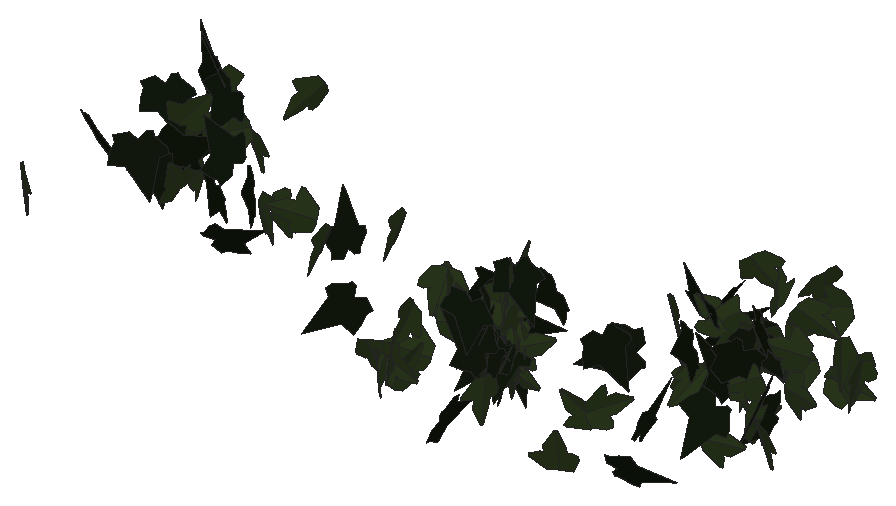
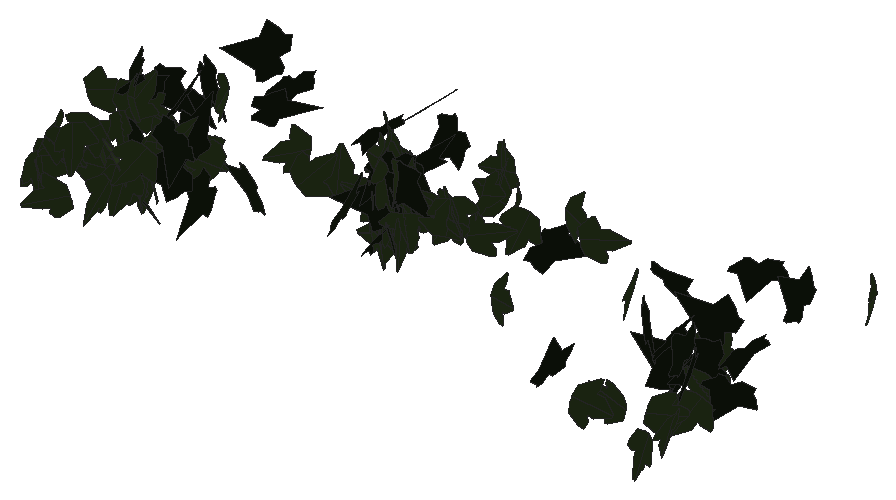
# SketchUp Ruby script. Lengths in inches.
U = 1.inch
M = Sketchup.active_model
def pt(a) = Geom::Point3d.new(a.map { |v| v * U })
def face(e, loops, mat)
  f = e.add_face(loops[0].map { |a| pt(a) })
  loops[1..].each { |l| e.add_face(l.map { |a| pt(a) }).erase! }
  f.material = f.back_material = mat if mat
  f
end
# faces: each face lists its corners as indices into pts; further lists are holes
def faces(e, pts, list, mat = nil) = list.each { |f| face(e, (f[0].is_a?(Array) ? f : [f]).map { |l| l.map { |i| pts[i] } }, mat) }
# xy, xz, yz: faces in a plane at the given z, y or x. An outline is a flat list of corners, or four numbers for a rectangle; further outlines are holes
def ring(l) = l.size == 4 ? [[l[0], l[1]], [l[2], l[1]], [l[2], l[3]], [l[0], l[3]]] : l.each_slice(2).to_a
def flat(e, list, mat, &to3) = list.each { |f| face(e, (f[0].is_a?(Array) ? f : [f]).map { |l| ring(l).map { |u, v| to3.(u, v) } }, mat) }
def xy(e, z, list, mat = nil) = flat(e, list, mat) { |x, y| [x, y, z] }
def xz(e, y, list, mat = nil) = flat(e, list, mat) { |x, z| [x, y, z] }
def yz(e, x, list, mat = nil) = flat(e, list, mat) { |y, z| [x, y, z] }
def lines(e, pts, list) = list.each { |a, b| e.add_line(pt(pts[a]), pt(pts[b])) }
# prism: a flat outline (further loops are holes) pulled along v
def prism(e, loops, v, mat = nil)
  f = face(e, loops, mat); d = Geom::Vector3d.new(v.map { |x| x * U })
  f.pushpull(f.normal.samedirection?(d) ? d.length : -d.length)
end
def box(e, o, s, mat = nil) = prism(e, [[o, [o[0] + s[0], o[1], o[2]], [o[0] + s[0], o[1] + s[1], o[2]], [o[0], o[1] + s[1], o[2]]]], [0, 0, s[2]], mat)
def at(x, y, z, deg = 0) = Geom::Transformation.translation(pt([x, y, z])) * Geom::Transformation.rotation(ORIGIN, Z_AXIS, deg.degrees)
def axes(o, x, y, z) = Geom::Transformation.new([*x, 0, *y, 0, *z, 0, *pt(o).to_a, 1])
def part(name) = M.definitions.add(name)
# library, detail: a bought-in or finely detailed component or shape, given as its bounding box
def library(name, o, s) = part(name).tap { |d| box(d.entities, o, s) }
def detail(e, o, s) = box(e.add_group.entities, o, s)
def put(e, d, t, mat = nil) = e.add_instance(d, t).tap { |i| i.material = mat if mat }
def group(e, t, mat = nil) = e.add_group.tap { |g| g.transformation = t; g.material = mat if mat }.entities
root = M.entities
M.materials.add("efeu1").color = [18, 25, 13]
M.materials.add("efeu2").color = [43, 57, 29]
c1 = part("ivyleaf_9")
p = [[1.54,2.16,1.25],[1.36,2.04,1.19],[-0.21,0.99,0.68],[-0.71,1.11,0.82],[-0.85,0.86,0.67],[-0.8,0.17,0.21],
  [-0.9,-0.01,0.1],[-0.67,-0.16,-0.02],[-0.08,-0.08,-0.05],[-0.03,-0.6,-0.4],[0.65,-0.88,-0.66],[0.83,-0.6,-0.49],
  [1.29,-0.42,-0.43],[1.8125,-0.07,-0.26],[1.21,0.44,0.15]]
faces(c1.entities,p,[[0,1,2,3,4,5,6,7,8,9,10,11,12,13,14]],"efeu1")
c2 = part("ivyleaf_10")
p = [[0,0.5,-0.03],[-0.0625,2.02,-0.43],[-0.19,2.01,-0.46],[-0.54,1.05,-0.29],[-0.52,0.625,-0.18],[-0.83,0.76,-0.28],
  [-1.16,0.64,-0.33],[-1.15,0.33,-0.24],[-0.77,-0.39,0.02],[-0.3,-0.51,0.16],[0.04,-0.48,0.23],[-0.02,2.01,-0.4375],
  [-0.06,2.01,-0.43],[0.04,-0.49,0.23],[0.67,-0.49,0.14],[1.38,0.36,-0.2],[1.375,0.51,-0.24],[0.81,0.65,-0.19],
  [0.62,0.59,-0.15],[0.6,1.09,-0.28],[0.5,1.23,-0.31]]
faces(c2.entities,p,[[0,1,2,3,4,5,6,7,8,9,10],[11,12,0,13,14,15,16,17,18,19,20]],"efeu2")
p = [[2445.43,81.9375,196.9],[2445.43,81.9375,197.07]]
lines(root,p,[[0,1]])
put(root,c1,axes([33.99,224.77,197.71],[-0.20049,-0.2567,-0.37935],[0.23865,0.29491,-0.32569],[0.39096,-0.31166,0.00427]))
put(root,c2,axes([34.07,219.18,197.74],[-0.16659,0.29333,-0.36906],[0.17893,-0.3228,-0.33732],[-0.43616,-0.24446,0.00258]))
put(root,c2,axes([34.48,226.46,197.29],[-0.09335,0.48943,0.04172],[-0.0077,0.041,-0.49826],[-0.49115,-0.09367,-0.00012]))
put(root,c1,axes([34.73,225.63,197.8],[0.01209,-0.36749,0.33883],[0.04185,0.33848,0.36562],[-0.4981,0.01952,0.03894]))
put(root,c2,axes([34.67,224.69,197.0625],[-0.30662,-0.27661,0.2819],[0.21392,0.18368,0.41292],[-0.332,0.37383,0.0057]))
put(root,c1,axes([34.625,221.24,198.21],[0.16375,-0.23934,0.40731],[0.25037,-0.3216,-0.28963],[0.40063,0.29881,0.01452]))
put(root,c2,axes([34.95,224.96,196.9375],[-0.4166,-0.11879,-0.24967],[0.24274,0.05905,-0.43312],[0.13239,-0.48208,0.00847]))
put(root,c1,axes([34.84,225.55,198.51],[0.12113,-0.28375,0.39346],[0.16463,-0.35743,-0.30845],[0.45632,0.20427,0.00684]))
put(root,c2,axes([35.65,225.55,196.75],[0.09653,0.05092,-0.48794],[-0.41929,-0.24963,-0.109],[-0.25471,0.43022,-0.00549]))
put(root,c1,axes([35.25,222.67,197.35],[0.02822,-0.47968,-0.13825],[-0.0084,0.13799,-0.48051],[0.49913,0.02944,-0.00027]))
put(root,c2,axes([35.52,226.22,196.24],[-0.43482,0.24661,-0.01067],[0.00928,-0.00527,-0.49989],[-0.24667,-0.43492,0]))
put(root,c1,axes([35.72,223.19,196.98],[0.18169,0.22407,0.40839],[0.25017,0.32283,-0.28843],[-0.39294,0.30915,0.0052]))
put(root,c1,axes([35.97,224.77,198.23],[-0.08125,-0.41344,0.2692],[-0.03869,-0.26665,-0.42119],[0.49183,-0.08928,0.01134]))
put(root,c2,axes([36.18,222.52,196.71],[-0.08016,-0.41395,-0.26873],[-0.05032,-0.26398,0.42164],[-0.49096,0.09464,0.00066]))
put(root,c1,axes([36.2,220.94,198.6],[-0.1834,-0.35628,-0.29904],[0.13765,0.26548,-0.40072],[0.44431,-0.22931,0.0007]))
put(root,c1,axes([36.04,222.55,197.57],[0.02202,-0.03544,0.49826],[0.48158,-0.13095,-0.0306],[0.13266,0.48125,0.02837]))
put(root,c2,axes([36.56,222.84,197.14],[0.27013,-0.2979,-0.29713],[-0.18839,0.23009,-0.40196],[0.37622,0.32911,0.01207]))
put(root,c2,axes([36.63,227.24,197.46],[-0.04899,-0.28397,0.40861],[-0.07582,-0.40153,-0.28814],[0.49178,-0.09019,-0.00373]))
put(root,c1,axes([36.75,223.21,196.58],[0.24788,-0.1426,-0.41015],[0.35342,-0.20814,0.28596],[-0.25229,-0.43167,-0.00239]))
put(root,c1,axes([38.01,222.26,198.14],[-0.44625,-0.03571,-0.22268],[-0.22058,-0.03372,0.44745],[-0.04698,0.49758,0.01434]))
put(root,c1,axes([37.62,222.24,195.85],[0.35713,0.26788,-0.22516],[0.18021,0.13499,0.44643],[0.29997,-0.40002,-0.00014]))
put(root,c1,axes([38.4,222.59,197.26],[-0.00087,0.02944,-0.49913],[-0.49516,0.0692,0.00494],[0.06937,0.49431,0.02903]))
put(root,c2,axes([37.75,224.46,195.75],[0.07346,-0.02372,-0.49401],[0.45875,-0.18335,0.07702],[-0.1848,-0.46457,-0.00517]))
put(root,c2,axes([39.3125,221.87,197.47],[-0.22943,0.43794,0.07465],[-0.03636,0.06522,-0.49439],[-0.44277,-0.23228,0.00191]))
put(root,c1,axes([40.07,224.18,195.7],[-0.18193,-0.32901,0.32963],[0.16047,0.28793,0.37596],[-0.43721,0.24258,0.00082]))
put(root,c2,axes([40.88,221.59,197.93],[0.07067,0.05309,0.49213],[-0.4077,-0.27565,0.08828],[0.28068,-0.41376,0.00433]))
put(root,c2,axes([41.82,223.99,197.03],[0.1284,-0.27823,0.3951],[0.18079,-0.35146,-0.30625],[0.44814,0.22151,0.01035]))
put(root,c2,axes([41.92,220.97,198.01],[0.14855,-0.35812,0.31573],[0.11556,-0.29386,-0.38768],[0.46323,0.18815,-0.00454]))
put(root,c1,axes([42.96,220.74,196.73],[-0.00313,-0.06102,-0.49625],[0.0235,-0.49573,0.06081],[-0.49944,-0.02294,0.00597]))
put(root,c2,axes([44.44,219.68,196.38],[-0.47888,0.01544,-0.14294],[0.14287,-0.00437,-0.47913],[-0.01604,-0.49974,-0.00023]))
put(root,c2,axes([45.22,220.58,196.09],[0.09156,0.1105,0.47896],[-0.36216,-0.31425,0.14173],[0.33235,-0.37288,0.02249]))
put(root,c2,axes([44.97,221.82,197.57],[0.43259,0.22116,-0.11814],[-0.10696,-0.05032,-0.48583],[-0.22678,0.4456,0.00377]))
put(root,c2,axes([45.07,221.89,196.87],[0.45483,0.20045,0.05436],[-0.05059,-0.02001,0.49703],[0.20143,-0.45763,0.00208]))
put(root,c2,axes([45.05,220.41,197.24],[0.03378,0.26659,-0.42165],[-0.04632,-0.41911,-0.2687],[-0.4967,0.05721,-0.00362]))
put(root,c2,axes([44.91,221.86,197.36],[0.26708,-0.09961,0.41079],[0.38407,-0.14574,-0.28504],[0.17653,0.4678,-0.00134]))
put(root,c2,axes([45.58,218.57,196.31],[0.17425,-0.11294,0.45484],[-0.38747,0.23827,0.2076],[-0.26364,-0.42482,-0.00449]))
put(root,c2,axes([45.08,221.85,197.05],[0.40454,0.026,0.29269],[0.29195,0.02092,-0.40538],[-0.03333,0.49889,0.00174]))
put(root,c2,axes([45.75,219.05,196.24],[0.01248,-0.3883,0.31475],[-0.01628,0.31437,0.38847],[-0.49958,-0.01995,-0.00479]))
put(root,c2,axes([45.65,219.02,197.15],[-0.02808,0.1309,-0.48174],[0.13539,-0.46242,-0.13354],[-0.4805,-0.13795,-0.00947]))
put(root,c2,axes([45.58,221.15,196.89],[0.14192,-0.01278,-0.47927],[0.47823,-0.0316,0.14246],[-0.03393,-0.49884,0.00326]))
put(root,c2,axes([45.67,218.72,196.92],[0.10422,-0.00058,0.48902],[0.48465,0.06677,-0.10321],[-0.06518,0.49552,0.01448]))
put(root,c1,axes([46.59,221.88,197.81],[0.02511,0.0789,-0.4931],[-0.42305,-0.25896,-0.06298],[-0.26532,0.42037,0.05375]))
put(root,c2,axes([46.4,221.96,196.47],[0.06898,-0.41485,-0.27045],[-0.03862,0.26773,-0.42051],[0.49371,0.0789,0.00489]))
put(root,c2,axes([46.27,221.97,196.76],[0.45481,0.20754,-0.00875],[-0.00913,-0.00107,-0.49992],[-0.20753,0.45489,0.00282]))
put(root,c2,axes([46.61,221.9,197.77],[-0.01187,0.04,0.49826],[-0.36347,0.34145,-0.03607],[-0.34314,-0.36306,0.02097]))
put(root,c2,axes([46.91,221.51,196.81],[-0.10626,0.04987,0.48603],[-0.48511,0.0484,-0.11103],[-0.05812,-0.49515,0.03809]))
put(root,c2,axes([46.95,221.56,195.97],[-0.21155,-0.15711,-0.42493],[-0.31152,-0.29006,0.26234],[-0.32894,0.37574,0.02484]))
put(root,c2,axes([46.9,221.8125,197.45],[-0.09614,-0.4741,0.12643],[-0.02558,-0.12382,-0.48375],[0.49,-0.09948,-0.00044]))
put(root,c2,axes([46.96,222,198.11],[0.17186,-0.31559,0.34766],[-0.15837,0.30956,0.35929],[-0.44202,-0.23361,0.00644]))
put(root,c1,axes([47.09,220.72,197.44],[-0.36926,0.28841,-0.17456],[0.13773,-0.10724,-0.46854],[-0.3077,-0.39411,-0.00024]))
put(root,c1,axes([46.85,221.41,196.47],[0.4271,-0.25983,0.0085],[-0.00579,0.00684,0.49992],[-0.25991,-0.42713,0.00283]))
put(root,c2,axes([46.91,221.67,196.4],[-0.03568,-0.43554,0.24296],[0.15476,-0.24123,-0.40971],[0.47411,0.04596,0.15203]))
put(root,c1,axes([46.83,221.74,198.1],[0.044,-0.27449,-0.41559],[-0.03803,0.41414,-0.27756],[0.49661,0.05604,0.01557]))
put(root,c1,axes([47.27,220.93,196.22],[-0.48391,0.04274,-0.11835],[-0.11789,0.01046,0.48579],[0.044,0.49806,-0.00004]))
put(root,c1,axes([46.96,221.82,196.36],[-0.29356,0.09067,-0.39447],[0.38112,-0.10216,-0.3071],[-0.13628,-0.48098,-0.00913]))
put(root,c1,axes([47.27,220.8,196.86],[-0.49686,0.02635,-0.04936],[0.04919,-0.00452,-0.49755],[-0.02666,-0.49928,0.0019]))
put(root,c2,axes([47.15,221.5,198.25],[0.04516,-0.07712,-0.49195],[-0.03689,0.49209,-0.08053],[0.49659,0.04357,0.03876]))
put(root,c2,axes([46.85,221.77,196.98],[0.37202,-0.23035,-0.24195],[0.20387,-0.13034,0.43755],[-0.26465,-0.42421,-0.00305]))
put(root,c2,axes([47.16,220.59,196.28],[0.11955,-0.42379,-0.23688],[-0.04635,0.23288,-0.44002],[0.48328,0.12717,0.01639]))
put(root,c1,axes([46.93,222,196.2],[0.13753,-0.47985,-0.02873],[-0.00676,0.02795,-0.49917],[0.48067,0.13769,0.0012]))
put(root,c2,axes([46.81,221.33,197.8],[0.09021,0.07129,0.4866],[0.38878,0.29263,-0.11495],[-0.30118,0.39911,-0.00263]))
put(root,c1,axes([47.4,220.23,197.04],[-0.23992,-0.4382,-0.02037],[-0.00473,-0.02063,0.49955],[-0.43865,0.2399,0.00576]))
put(root,c1,axes([47.18,221.42,196.68],[-0.28672,-0.39019,-0.12467],[0.08252,0.09404,-0.48409],[0.40122,-0.29818,0.01047]))
put(root,c1,axes([47.08,223.43,197.22],[0.29696,-0.29961,-0.26842],[0.18716,-0.19243,0.42183],[-0.35607,-0.35101,-0.00214]))
put(root,c1,axes([46.91,221.82,197.04],[0.1811,0.16326,-0.43652],[0.24958,0.36153,0.23876],[0.39359,-0.30437,0.04945]))
put(root,c2,axes([47.14,221.45,198.69],[0.38973,-0.21916,0.22378],[0.19876,-0.10303,-0.44708],[0.24208,0.43744,0.00681]))
put(root,c2,axes([47.36,221.6875,196.02],[0.14489,-0.47723,-0.03556],[-0.01071,0.03391,-0.49873],[0.47843,0.14528,-0.0004]))
put(root,c2,axes([47.36,221.64,197.69],[0.05273,-0.47094,-0.15949],[0.0517,0.16471,-0.46925],[0.49452,0.033,0.06606]))
put(root,c2,axes([47.1,221.73,196.87],[0.3853,-0.04576,0.31535],[0.31589,-0.01026,-0.38744],[0.04193,0.4978,0.021]))
put(root,c2,axes([47.39,220.3,196.09],[-0.06669,-0.48911,0.07952],[0.11637,-0.09345,-0.47721],[0.48168,-0.04515,0.1263]))
put(root,c2,axes([47.4,221.57,196.52],[0.06504,-0.49472,-0.03202],[0.08465,0.0429,-0.49091],[0.48847,0.05844,0.08934]))
put(root,c2,axes([47.08,221.66,195.93],[-0.15529,0.04413,-0.47322],[0.45349,-0.13524,-0.16143],[-0.14224,-0.47934,0.00198]))
put(root,c1,axes([47.35,219.83,198.55],[-0.0669,-0.48137,0.11752],[0.11734,-0.1306,-0.46816],[0.48141,-0.03506,0.13044]))
put(root,c1,axes([47.37,221.59,198.75],[0.05284,-0.47518,-0.14634],[0.05204,0.15164,-0.4736],[0.49447,0.03482,0.06548]))
put(root,c2,axes([47.42,221.57,196.65],[0.15617,-0.00489,-0.47496],[0.47409,0.03225,0.15555],[0.02911,-0.49894,0.01471]))
put(root,c1,axes([48.23,217.6,196.59],[-0.13141,0.21377,-0.43248],[-0.2424,0.35829,0.25075],[0.4171,0.27556,0.00947]))
put(root,c2,axes([50.26,220.84,196],[-0.33796,-0.07188,-0.36141],[-0.34663,-0.10437,0.3449],[-0.12503,0.48367,0.02072]))
put(root,c2,axes([50.27,219.5625,195.29],[-0.46566,-0.1798,-0.02884],[-0.02691,-0.01037,0.49917],[-0.1801,0.46644,-0.00002]))
put(root,c2,axes([50.72,220.47,196.48],[-0.0099,-0.05584,0.49677],[0.0771,0.49076,0.0567],[-0.49392,0.07772,-0.0011]))
put(root,c1,axes([51.15,221.37,197.84],[-0.29176,-0.14244,0.38024],[-0.34342,-0.16326,-0.32467],[0.21665,-0.45062,-0.00257]))
put(root,c1,axes([50.8,220.67,198.4375],[0.05855,-0.39124,-0.30578],[-0.0289,0.30469,-0.39538],[0.49572,0.06398,0.01307]))
put(root,c1,axes([51.35,223.86,197.95],[0.30247,-0.26771,0.29469],[-0.17794,0.24016,0.40082],[-0.35616,-0.34735,0.05001]))
put(root,c1,axes([51.26,221.58,195.64],[-0.24802,0.43391,0.01435],[-0.00203,-0.01768,0.49968],[0.43415,0.2478,0.01053]))
put(root,c1,axes([51.31,223.37,196.45],[0.46195,-0.06338,-0.18052],[-0.176,0.04423,-0.46591],[0.07503,0.49399,0.01855]))
put(root,c1,axes([51.65,224.08,198.14],[-0.00956,0.46699,0.17841],[-0.00036,0.17844,-0.46708],[-0.49991,-0.00906,-0.00307]))
put(root,c2,axes([51.39,225.85,198.46],[-0.38846,-0.13428,-0.28472],[0.26853,0.09467,-0.41101],[0.16428,-0.47224,-0.00144]))
put(root,c2,axes([51.43,222.54,198.76],[-0.26081,0.32793,-0.27283],[0.16213,-0.21959,-0.41892],[-0.39458,-0.30698,0.00821]))
put(root,c1,axes([51.5,224.13,197.33],[0.00592,0.38019,-0.32469],[-0.01092,0.32473,0.38004],[0.49985,0.00259,0.01215]))
put(root,c2,axes([51.81,224,197.77],[0.20186,0.35672,0.28637],[-0.1451,-0.24692,0.40985],[0.43382,-0.24857,0.00384]))
put(root,c2,axes([51.8,222.58,196.61],[-0.06708,-0.2934,0.39927],[0.08345,0.39047,0.30095],[-0.4884,0.10702,-0.00342]))
put(root,c2,axes([52.125,222.67,196.98],[0.30539,0.21412,-0.333],[-0.26979,-0.19523,-0.37296],[-0.28975,0.40747,-0.00371]))
put(root,c2,axes([52.28,225.56,197.8125],[0.30424,-0.01226,0.3966],[-0.327,0.27533,0.25936],[-0.22475,-0.41719,0.15951]))
put(root,c2,axes([52.33,224.12,197.77],[0.13748,0.22819,-0.42312],[-0.22238,-0.35998,-0.26639],[-0.4262,0.26143,0.00251]))
put(root,c1,axes([52.75,221.59,198.48],[0.02039,0.01375,-0.49939],[-0.49832,-0.03498,-0.02131],[-0.03552,0.49859,0.01228]))
put(root,c2,axes([52.51,225.85,197.13],[-0.00267,0.2682,0.42198],[-0.14442,0.40358,-0.25742],[-0.47868,-0.12326,0.07531]))
put(root,c2,axes([52.24,224.68,196.54],[-0.21701,0.12993,0.4313],[0.37818,-0.20753,0.2528],[0.24472,0.43594,-0.0082]))
put(root,c2,axes([52.68,224.84,196.97],[-0.46867,-0.15175,-0.08556],[0.08224,0.02377,-0.49262],[0.15357,-0.47582,0.00268]))
put(root,c2,axes([52.52,223.84,196.39],[0.04406,-0.05632,0.49486],[0.43039,-0.2457,-0.06628],[0.25064,0.43181,0.02683]))
put(root,c2,axes([53.05,222.91,197.02],[-0.00918,0.00141,0.49991],[-0.08392,0.4929,-0.00293],[-0.49282,-0.08396,-0.00881]))
put(root,c1,axes([53.26,222.27,197.39],[-0.03603,-0.46882,0.17002],[0.01212,0.16959,0.4702],[-0.49855,0.038,-0.00086]))
put(root,c2,axes([53.22,226.13,198.54],[-0.14737,-0.46765,-0.09789],[0.01154,0.09893,-0.48998],[0.47765,-0.14668,-0.01836]))
put(root,c2,axes([53.46,224.04,197.86],[-0.39683,0.15581,0.26124],[-0.26695,0.02746,-0.42188],[-0.14581,-0.47431,0.06139]))
put(root,c2,axes([53.28,223.27,195.87],[-0.0129,-0.04148,-0.49811],[0.13856,0.47845,-0.04343],[0.48024,-0.13915,-0.00085]))
put(root,c2,axes([53.59,223.46,198.04],[-0.30818,-0.2153,-0.32965],[-0.23354,-0.23707,0.37317],[-0.31699,0.38399,0.04556]))
put(root,c2,axes([53.73,224.79,196.98],[0.1377,0.07041,-0.47548],[-0.44545,-0.16713,-0.15375],[-0.18059,0.46595,0.0167]))
put(root,c1,axes([53.71,223.52,196.09],[-0.43454,0.24564,-0.02894],[0.02478,-0.01497,-0.49916],[-0.2461,-0.43524,0.00083]))
put(root,c1,axes([53.64,222.44,198.25],[0.03369,0.1346,-0.48036],[-0.083,-0.47323,-0.13842],[-0.49191,0.08907,-0.00955]))
put(root,c2,axes([53.8125,222.63,197.52],[-0.19961,-0.06208,0.4542],[-0.37514,-0.26262,-0.20076],[0.26349,-0.42092,0.05826]))
put(root,c2,axes([53.88,226.02,198.05],[0.20515,-0.05925,-0.45211],[-0.44223,0.09497,-0.21311],[0.11113,0.48731,-0.01344]))
put(root,c1,axes([53.73,221.24,197.27],[-0.45752,-0.19345,-0.05703],[0.05233,0.02266,-0.49674],[0.19477,-0.4605,-0.00049]))
put(root,c2,axes([53.24,221.76,196],[0.02785,-0.01405,-0.49903],[0.49065,-0.09146,0.02996],[-0.09213,-0.49136,0.0087]))
put(root,c2,axes([53.48,223.46,198.29],[0.1264,-0.21997,0.43085],[0.23639,-0.36045,-0.25337],[0.42207,0.26775,0.01288]))
put(root,c1,axes([53.48,223.02,198.49],[0.0671,-0.32015,-0.37815],[-0.02922,0.37838,-0.32553],[0.49462,0.06578,0.03207]))
put(root,c2,axes([53.59,224.58,197.61],[0.21992,-0.39228,0.21853],[0.10876,-0.18955,-0.44971],[0.43567,0.24534,0.00196]))
put(root,c2,axes([53.49,225.1,198.14],[-0.29212,-0.04973,-0.40273],[0.40224,0.03002,-0.29547],[0.05356,-0.49661,0.02247]))
put(root,c1,axes([53.73,222.95,198.89],[0.35047,-0.15677,-0.3203],[-0.28617,0.14432,-0.38377],[0.21278,0.45232,0.01143]))
put(root,c1,axes([53.97,222.96,197.07],[-0.32778,0.20889,-0.31452],[0.25181,-0.1894,-0.38823],[-0.28133,-0.41291,0.01896]))
put(root,c1,axes([53.51,217.91,196.97],[0.31927,-0.09839,0.372],[0.37596,-0.02318,-0.32881],[0.08194,0.48968,0.05918]))
put(root,c2,axes([54.07,222.67,196.1],[-0.41647,0.27553,-0.02528],[0.01954,-0.01629,-0.49935],[-0.27599,-0.41692,0.0028]))
put(root,c2,axes([53.82,224.17,196.52],[0.00311,-0.01273,-0.49983],[0.42853,-0.25744,0.00922],[-0.25759,-0.42844,0.00931]))
put(root,c2,axes([54.6,223.48,198.09],[0.08663,0.06926,0.48754],[-0.3977,-0.28209,0.11074],[0.2904,-0.40697,0.00622]))
put(root,c2,axes([54.08,225.55,196.23],[0.11844,0.09318,0.47675],[0.37311,0.29678,-0.1507],[-0.31106,0.39146,0.00077]))
put(root,c2,axes([54.68,225.51,196.84],[-0.31032,-0.38729,0.06092],[0.02643,-0.09818,-0.48955],[0.39116,-0.30061,0.0814]))
put(root,c2,axes([54.74,225.53,196.99],[-0.1571,-0.47203,0.05008],[0.0575,-0.07129,-0.49154],[0.47118,-0.14868,0.07668]))
put(root,c2,axes([54.76,224.92,197.67],[-0.06023,0.46409,-0.17604],[0.0113,-0.17601,-0.46786],[-0.49623,-0.06033,0.01071]))
put(root,c2,axes([54.95,225.3,196.95],[0.21857,-0.39449,0.21588],[0.12643,-0.17644,-0.45043],[0.43156,0.25148,0.02262]))
